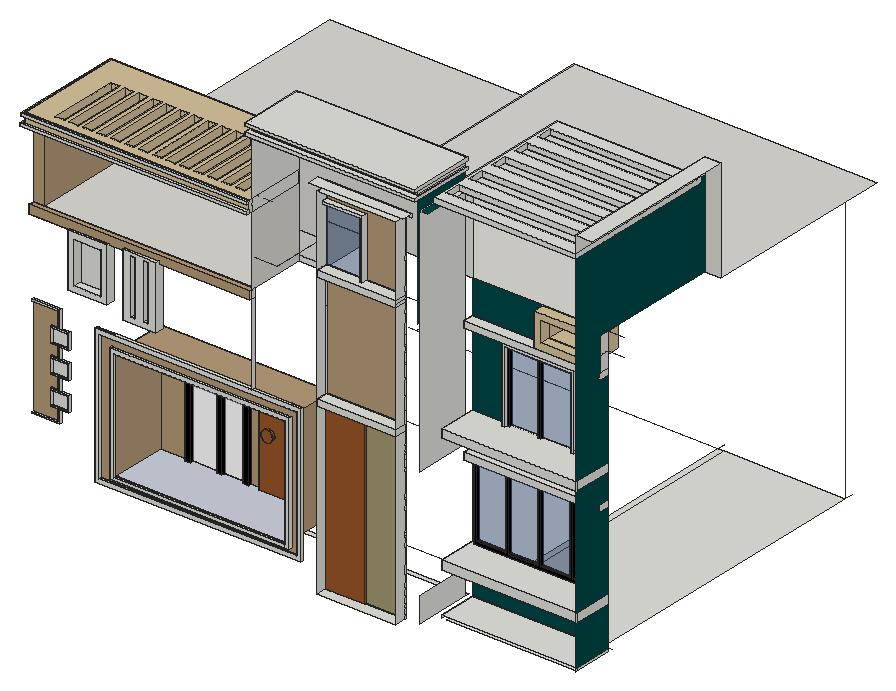
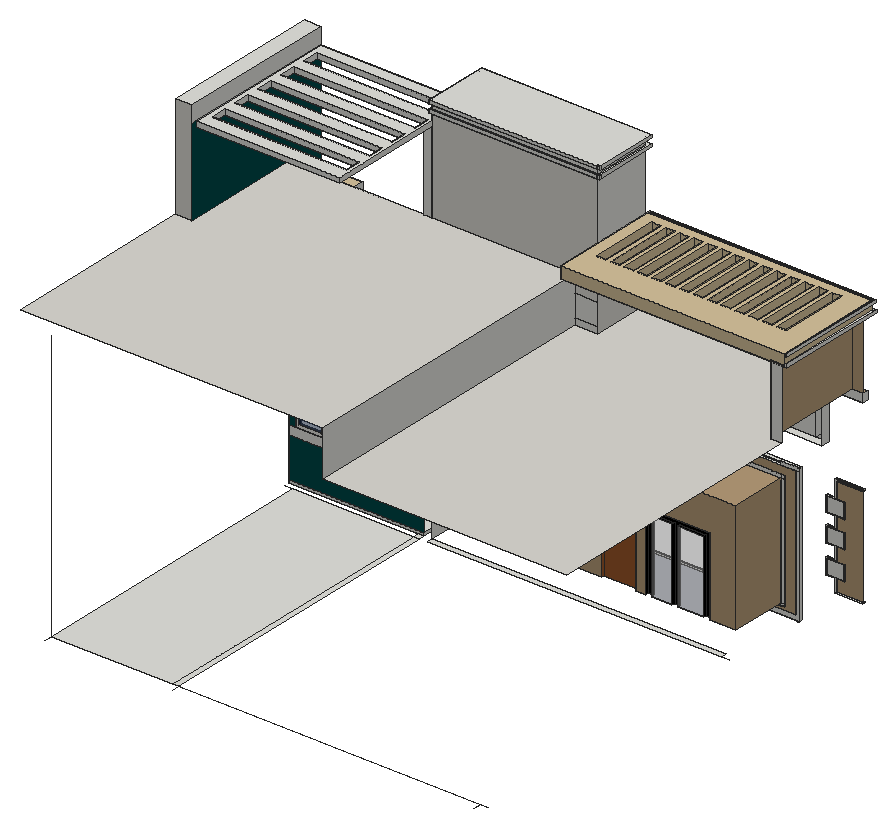
# SketchUp Ruby script. Lengths in inches.
U = 1.inch
M = Sketchup.active_model
def pt(a) = Geom::Point3d.new(a.map { |v| v * U })
def face(e, loops, mat)
  f = e.add_face(loops[0].map { |a| pt(a) })
  loops[1..].each { |l| e.add_face(l.map { |a| pt(a) }).erase! }
  f.material = f.back_material = mat if mat
  f
end
# faces: each face lists its corners as indices into pts; further lists are holes
def faces(e, pts, list, mat = nil) = list.each { |f| face(e, (f[0].is_a?(Array) ? f : [f]).map { |l| l.map { |i| pts[i] } }, mat) }
# xy, xz, yz: faces in a plane at the given z, y or x. An outline is a flat list of corners, or four numbers for a rectangle; further outlines are holes
def ring(l) = l.size == 4 ? [[l[0], l[1]], [l[2], l[1]], [l[2], l[3]], [l[0], l[3]]] : l.each_slice(2).to_a
def flat(e, list, mat, &to3) = list.each { |f| face(e, (f[0].is_a?(Array) ? f : [f]).map { |l| ring(l).map { |u, v| to3.(u, v) } }, mat) }
def xy(e, z, list, mat = nil) = flat(e, list, mat) { |x, y| [x, y, z] }
def xz(e, y, list, mat = nil) = flat(e, list, mat) { |x, z| [x, y, z] }
def yz(e, x, list, mat = nil) = flat(e, list, mat) { |y, z| [x, y, z] }
def lines(e, pts, list) = list.each { |a, b| e.add_line(pt(pts[a]), pt(pts[b])) }
# prism: a flat outline (further loops are holes) pulled along v
def prism(e, loops, v, mat = nil)
  f = face(e, loops, mat); d = Geom::Vector3d.new(v.map { |x| x * U })
  f.pushpull(f.normal.samedirection?(d) ? d.length : -d.length)
end
def box(e, o, s, mat = nil) = prism(e, [[o, [o[0] + s[0], o[1], o[2]], [o[0] + s[0], o[1] + s[1], o[2]], [o[0], o[1] + s[1], o[2]]]], [0, 0, s[2]], mat)
def at(x, y, z, deg = 0) = Geom::Transformation.translation(pt([x, y, z])) * Geom::Transformation.rotation(ORIGIN, Z_AXIS, deg.degrees)
def axes(o, x, y, z) = Geom::Transformation.new([*x, 0, *y, 0, *z, 0, *pt(o).to_a, 1])
def part(name) = M.definitions.add(name)
# library, detail: a bought-in or finely detailed component or shape, given as its bounding box
def library(name, o, s) = part(name).tap { |d| box(d.entities, o, s) }
def detail(e, o, s) = box(e.add_group.entities, o, s)
def put(e, d, t, mat = nil) = e.add_instance(d, t).tap { |i| i.material = mat if mat }
def group(e, t, mat = nil) = e.add_group.tap { |g| g.transformation = t; g.material = mat if mat }.entities
root = M.entities
M.materials.add("[0034_Wheat]").color = [214, 194, 156]
M.materials.add("[0035_Tan]").color = [181, 155, 120]
M.materials.add("[0079_Teal]").color = [0, 71, 71]
M.materials.add("[0137_Black]").color = [0, 0, 0]
M.materials.add("[Marble Carrara Floor Tile]").color = [204, 208, 219]
M.materials.add("[Terrazzo Tile Light]").color = [219, 217, 210]
M.materials.add("[Translucent Glass Blue]").color = [52, 78, 124]
M.materials["[Translucent Glass Blue]"].alpha = 0.5
M.materials.add("[Translucent Glass Gray]").color = [201, 201, 201]
M.materials["[Translucent Glass Gray]"].alpha = 0.5
M.materials.add("[Wood Cherry Original]").color = [152, 86, 42]
M.materials.add("[Wood Lumber ButtJoined]").color = [164, 152, 112]
xy(root,120,[[437.125,271.56,577.1875,313.125],[106.1875,313.125,423.03,319.125],[431.125,313.125,437.125,319.125],[431.125,319.125,437.125,643.9375],[437.125,319.125,568.1875,643.9375]])
xy(root,121,[[323.96,237.8125,409.46,237.8125,409.46,249.8125,366.71,249.8125,366.71,248.8125,323.96,248.8125],[323.96,248.8125,366.71,249.8125],[323.96,249.8125,366.71,250.75],[366.71,249.8125,409.46,250.75]])
xy(root,123,[[431.125,271.56,577.1875,313.125]])
xy(root,136.125,[[74.71,249.8125,296.54,252.8125],[74.71,252.8125,296.54,253.5]])
xy(root,140.43,[[79.1,249.8125,292.23,252.8125]])
xy(root,144.1875,[[91.02,249.8125,284.58,252.8125]])
xy(root,147.125,[[95.27,249.8125,279.28,252.8125]])
xy(root,147.27,[[95.27,252.8125,279.28,252.8125,279.28,313.125,239.67,313.125,239.67,310.125,203.67,310.125,203.67,313.125,192.46,313.125,192.46,310.125,186.46,310.125,186.46,313.125,164.08,313.125,164.08,310.125,158.08,310.125,158.08,313.125,129.71,313.125,129.71,310.125,123.71,310.125,123.71,313.125,95.27,313.125]],"[Marble Carrara Floor Tile]")
xy(root,166.28,[[431.125,271.56,577.1875,313.125]])
xy(root,176.29,[[431.125,271.56,577.1875,271.56,577.1875,313.125,569.6,313.125,569.6,310.125,435.12,310.125,435.12,313.125,431.125,313.125],[435.12,310.125,569.6,313.125]])
xy(root,177.18,[[6.1875,251.5,36.19,253.5]])
xy(root,178.93,[[6.1875,251.5,34.19,253.5]])
xy(root,179.29,[[438.12,310.125,470.05,313.125],[473.05,310.125,503.8,313.125],[506.8,310.125,538.43,313.125],[541.43,310.125,566.6,313.125]],"[0137_Black]")
xy(root,191.55,[[25.74,251.5,34.19,253.5],[36.19,251.5,46.11,253.5]])
xy(root,192.55,[[26.74,251.5,45.11,253.5]])
xy(root,207.43,[[26.74,251.5,45.11,253.5]])
xy(root,208.43,[[25.74,251.5,34.15,253.5],[36.19,251.5,46.11,253.5]])
xy(root,222.43,[[25.74,251.5,34.15,253.5],[36.19,251.5,46.11,253.5]])
xy(root,223.43,[[26.74,251.5,45.11,253.5]])
xy(root,225.27,[[129.71,310.125,158.08,313.125],[164.08,310.125,186.46,313.125]],"[0137_Black]")
xy(root,231.27,[[123.71,310.125,192.46,313.125]],"[0137_Black]")
xy(root,238.3,[[26.74,251.5,45.11,253.5]])
xy(root,239.3,[[25.74,251.5,34.15,253.5],[36.19,251.5,46.11,253.5]])
xy(root,239.64,[[203.67,310.125,239.67,313.125]],"[Wood Cherry Original]")
xy(root,251.74,[[25.74,251.5,34.15,253.5],[36.19,251.5,46.11,253.5]])
xy(root,252.74,[[26.74,251.5,45.11,253.5]])
xy(root,256.41,[[438.12,310.125,470.05,313.125],[473.05,310.125,503.8,313.125],[506.8,310.125,538.43,313.125],[541.43,310.125,566.6,313.125]],"[0137_Black]")
xy(root,259.41,[[431.125,301.125,431.125,313.125,435.12,313.125,435.12,310.125,569.6,310.125,569.6,313.125,577.1875,313.125,577.1875,301.125],[435.12,310.125,569.6,313.125]])
xy(root,267,[[95.27,249.8125,279.28,252.8125],[431.125,301.125,577.1875,313.125]])
xy(root,267,[[95.27,252.8125,279.28,313.125]],"[0035_Tan]")
xy(root,267.61,[[26.74,251.5,45.11,253.5]])
xy(root,268.61,[[25.74,251.5,34.15,253.5],[36.19,251.5,46.11,253.5]])
xy(root,271.125,[[91.02,249.8125,284.58,252.8125]])
xy(root,280.1875,[[79.1,249.8125,292.23,252.8125]])
xy(root,284.3125,[[74.71,249.8125,243.98,249.8125,243.98,253.5,95.27,253.5,95.27,252.8125,74.71,252.8125],[243.98,249.8125,296.54,252.8125],[74.71,252.8125,95.27,253.5]])
xy(root,285.5,[[6.1875,251.5,34.15,253.5]])
xy(root,287.35,[[6.1875,251.5,36.19,253.5]])
xy(root,293.48,[[431.125,271.56,577.1875,313.125]])
xy(root,301.91,[[323.96,237.8125,323.96,248.8125,366.71,248.8125,366.71,250.75,409.46,250.75,409.46,237.8125],[323.96,248.8125,366.71,250.75]])
xy(root,303.01,[[431.125,271.56,577.1875,271.56,577.1875,313.125,545.36,313.125,545.36,307.125,542.36,307.125,542.36,310.125,539.8,310.125,539.8,313.125,507.6,313.125,507.6,310.125,504.6,310.125,504.6,313.125,473.54,313.125,473.54,310.125,470.98,310.125,470.98,307.125,467.98,307.125,467.98,313.125,431.125,313.125],[467.98,307.125,470.98,313.125],[542.36,307.125,545.36,313.125],[470.98,310.125,473.54,313.125],[504.6,310.125,507.6,313.125],
  [539.8,310.125,542.36,313.125]])
xy(root,306.52,[[109.1875,244.5,145.3125,253.5]])
xy(root,308.55,[[323.96,237.8125,409.46,250.75]])
xy(root,312.27,[[118.125,244.5,122.875,253.5],[131.8125,244.5,136,253.5]])
xy(root,314.76,[[50.28,244.5,92.36,253.5]])
xy(root,321.06,[[56.57,244.5,86.07,253.5]])
xy(root,366,[[56.57,244.5,86.07,253.5]])
xy(root,371.77,[[118.125,244.5,122.875,253.5],[131.8125,244.5,136,253.5],[50.28,247.5,92.36,253.5],[145,247.5,145.3125,253.5]])
xy(root,371.77,[[6.1875,247.5,50.28,253.5],[92.36,247.5,109.1875,253.5],[145.3125,247.5,243.98,253.5]],"[0035_Tan]")
xy(root,372.77,[[50.28,244.5,92.36,247.5]])
xy(root,374.77,[[109.1875,244.5,145.3125,247.5]])
xy(root,377.44,[[473.54,310.125,504.6,313.125],[507.6,310.125,539.8,313.125]],"[0137_Black]")
xy(root,380,[[470.98,307.125,542.36,310.125]])
xy(root,380.6875,[[6.1875,247.5,243.98,253.5]],"[0035_Tan]")
xy(root,380.6875,[[17.6875,253.5,243.98,253.5,243.98,313.125,269.04,313.125,269.04,652.9375,6.1875,652.9375,6.1875,363.1875,17.6875,363.1875]],"[Terrazzo Tile Light]")
xy(root,383,[[467.98,307.125,545.36,313.125]])
xy(root,387,[[431.125,301.125,577.1875,313.125]])
xy(root,394.0625,[[431.125,301.125,577.1875,301.125,577.1875,301.875,506.79,301.875,506.79,313.125,431.125,313.125],[506.79,301.875,577.1875,313.125]])
xy(root,401.12,[[513.85,301.875,570.13,313.125],[513.85,313.125,570.13,335.6875]],"[0034_Wheat]")
xy(root,423.19,[[513.85,301.875,570.13,313.125],[513.85,313.125,570.13,335.6875]],"[0034_Wheat]")
xy(root,426.24,[[323.96,237.8125,409.46,250.75]])
xy(root,430.25,[[506.79,301.875,577.1875,313.125]],"[0034_Wheat]")
xy(root,430.25,[[269.04,313.125,577.1875,313.125,577.1875,443.1875,594.5625,443.1875,594.5625,652.9375,269.04,652.9375]],"[Terrazzo Tile Light]")
xy(root,433.05,[[323.96,237.8125,409.46,237.8125,409.46,250.75,367.11,250.75,367.11,244.875,364.11,244.875,364.11,250.75,323.96,250.75],[364.11,244.875,367.11,250.75]])
xy(root,456,[[[0,243.25,243.98,363.1875],[161.16,256.96,170.97,331.71],[26.72,256.96,36.53,331.71],[41.66,256.96,51.47,331.71],[56.6,256.96,66.41,331.71],[71.53,256.96,81.35,331.71],[86.47,256.96,96.28,331.71],[101.41,256.96,111.22,331.71],[116.35,256.96,126.16,331.71],[131.28,256.96,141.1,331.71],[146.22,256.96,156.03,331.71],[176.1,256.96,185.91,331.71],[191.03,256.96,200.85,331.71],[205.97,256.96,215.78,331.71],[220.91,256.96,230.72,331.71]]],"[0034_Wheat]")
xy(root,458.95,[[0,243.25,2.25,246.25],[2.25,243.25,243.98,246.25],[0,246.25,2.25,363.1875]])
xy(root,465.625,[[0.4375,243.25,0.4375,363.1875,2.25,363.1875,2.25,246.25,243.98,246.25,243.98,243.25]])
xy(root,468.57,[[0.4375,243.25,243.98,243.25,243.98,246.25,2.25,246.25,2.25,363.1875,0.4375,363.1875]])
xy(root,468.625,[[[2.25,246.25,243.98,363.1875],[161.16,256.96,170.97,331.71],[26.72,256.96,36.53,331.71],[41.66,256.96,51.47,331.71],[56.6,256.96,66.41,331.71],[71.53,256.96,81.35,331.71],[86.47,256.96,96.28,331.71],[101.41,256.96,111.22,331.71],[116.35,256.96,126.16,331.71],[131.28,256.96,141.1,331.71],[146.22,256.96,156.03,331.71],[176.1,256.96,185.91,331.71],[191.03,256.96,200.85,331.71],[205.97,256.96,215.78,331.71],[220.91,256.96,230.72,331.71]]],"[0034_Wheat]")
xy(root,494.21,[[323.96,244.875,364.11,250.75]])
xy(root,497.21,[[323.96,244.875,367.11,250.75]])
xy(root,509.47,[[323.96,237.8125,409.46,249.8125]])
xy(root,514.78,[[315.58,237.8125,416.24,249.8125],[323.96,249.8125,409.46,250.75]])
xy(root,518.125,[[[422.6875,270.3125,422.6875,438.125,577.1875,438.125,577.1875,270.3125,431.125,270.3125,431.125,283.49,570.77,283.49,570.77,300.68,431.125,300.68,431.125,313.125,423.03,313.125,423.03,270.3125],[426.33,314.3,570.77,331.49],[426.33,345.12,570.77,362.3],[426.33,375.93,570.77,393.12],[426.33,406.74,570.77,423.93]],[423.03,270.3125,431.125,270.3125,431.125,283.49,426.33,283.49,426.33,300.68,431.125,300.68,431.125,313.125,423.03,313.125],[426.33,283.49,431.125,300.68]])
xy(root,518.125,[[423.03,252.8125,431.125,270.3125]],"[0079_Teal]")
xy(root,523.8125,[[[422.6875,270.3125,577.1875,438.125],[426.33,283.49,570.77,300.68],[426.33,314.3,570.77,331.49],[426.33,345.12,570.77,362.3],[426.33,375.93,570.77,393.12],[426.33,406.74,570.77,423.93]]])
xy(root,531.41,[[241.23,243.8125,241.23,313.125,243.98,313.125,243.98,249.8125,423.03,249.8125,423.03,313.125,243.98,313.125,243.98,314.6875,425.03,314.6875,425.03,243.8125],[241.23,313.125,243.98,314.6875]])
xy(root,534.9375,[[241.23,243.8125,425.03,243.8125,425.03,314.6875,243.98,314.6875,243.98,313.125,423.03,313.125,423.03,249.8125,243.98,249.8125,243.98,313.125,241.23,313.125],[241.23,313.125,243.98,314.6875]])
xy(root,540.18,[[241.23,243.8125,241.23,313.125,243.98,313.125,243.98,249.8125,423.03,249.8125,423.03,313.125,243.98,313.125,243.98,314.5625,425.03,314.5625,425.03,243.8125],[241.23,313.125,243.98,314.5625]])
xy(root,541.5625,[[577.1875,270.3125,594.5625,443.1875]])
xy(root,543.75,[[241.23,243.8125,425.03,243.8125,425.03,314.5625,243.98,314.5625,243.98,313.125,241.23,313.125],[241.23,313.125,243.98,314.5625]])
xz(root,237.8125,[[323.96,301.91,409.46,308.55],[323.96,426.24,409.46,433.05]])
xz(root,243.25,[[0,456,243.98,458.95],[0.4375,465.625,243.98,468.57]])
xz(root,243.8125,[[241.23,531.41,425.03,534.9375],[241.23,540.18,425.03,543.75]])
xz(root,244.5,[[[109.1875,306.52,145.3125,374.77],[118.125,312.27,122.875,371.77],[131.8125,312.27,136,371.77]],[[50.28,314.76,92.36,372.77],[56.57,321.06,86.07,366]]])
xz(root,244.875,[[364.11,433.05,367.11,433.05,367.11,497.21,323.96,497.21,323.96,494.21,364.11,494.21]])
xz(root,246.25,[[2.25,465.625,243.98,468.57],[2.25,468.57,243.98,468.625]])
xz(root,246.25,[[2.25,458.95,243.98,465.625]],"[0034_Wheat]")
xz(root,247.5,[[50.28,371.77,92.36,372.77]])
xz(root,247.5,[[6.1875,371.77,50.28,371.77,50.28,372.77,92.36,372.77,92.36,371.77,109.1875,371.77,109.1875,374.77,145.3125,374.77,145.3125,371.77,243.98,371.77,243.98,380.6875,6.1875,380.6875]],"[0035_Tan]")
xz(root,248.8125,[[323.96,121,366.71,301.91]],"[Wood Cherry Original]")
xz(root,249.8125,[[[74.71,136.125,296.54,284.3125],[79.1,140.43,292.23,280.1875]],[[91.02,144.1875,284.58,271.125],[95.27,147.125,279.28,267]],[323.96,509.47,409.46,514.78],[409.46,510.78,416.24,514.78],[243.98,531.37,423.03,531.41],
  [243.98,531.41,423.03,534.9375],[243.98,534.9375,423.03,540.18]])
xz(root,250.75,[[323.96,121,366.71,301.91],[323.96,301.91,409.46,308.55],[323.96,426.24,409.46,429.68],[323.96,429.68,323.96,430.05,367.11,430.05,367.11,433.05,409.46,433.05,409.46,429.68],[320.96,430.05,323.96,497.21],
  [323.96,430.05,367.11,433.05]])
xz(root,250.75,[[323.96,308.55,409.46,426.24],[367.11,433.05,409.46,433.05,409.46,514.78,323.96,514.78,323.96,497.21,367.11,497.21]],"[0035_Tan]")
xz(root,250.75,[[323.96,433.05,364.11,494.21]],"[Translucent Glass Blue]")
xz(root,250.75,[[366.71,121,409.46,301.91]],"[Wood Lumber ButtJoined]")
xz(root,251.5,[[6.1875,177.18,36.19,177.18,36.19,191.55,34.19,191.55,34.19,178.93,6.1875,178.93],[[25.74,191.55,46.11,208.43],[26.74,192.55,45.11,207.43]],[34.15,208.43,36.19,222.43],[[25.74,222.43,46.11,239.3],[26.74,223.43,45.11,238.3]],[34.15,239.3,36.19,251.74],
  [[25.74,251.74,46.11,268.61],[26.74,252.74,45.11,267.61]],[34.15,268.61,36.19,268.61,36.19,287.35,6.1875,287.35,6.1875,285.5,34.15,285.5]])
xz(root,252.8125,[[74.71,136.125,296.54,136.125,296.54,139.43,292.23,139.43,292.23,140.43,79.1,140.43,79.1,280.1875,74.71,280.1875],[292.23,139.43,296.54,147.27],[91.02,144.1875,95.27,145.0625],[95.27,144.1875,279.28,145.0625],[279.28,144.1875,284.58,147.27],
  [91.02,145.0625,95.27,147.125],[95.27,145.0625,279.28,147.125],[91.02,147.125,95.27,267],[95.27,147.125,279.28,147.27],[279.28,147.27,284.58,267],
  [292.23,147.27,296.54,267],[91.02,267,95.27,271.125],[95.27,267,284.58,271.125],[292.23,267,296.54,280.1875],[74.71,280.1875,95.27,284.3125],
  [284.58,280.1875,296.54,284.3125]])
xz(root,252.8125,[[[79.1,140.43,292.23,280.1875],[91.02,144.1875,284.58,271.125]]],"[0035_Tan]")
xz(root,253.5,[[26.74,192.55,45.11,207.43],[26.74,223.43,45.11,238.3],[26.74,252.74,45.11,267.61],[109.1875,312.27,118.125,371.77],[118.125,312.27,122.875,371.77],
  [122.875,312.27,131.8125,371.77],[131.8125,312.27,136,371.77],[136,312.27,145,371.77],[56.57,321.06,86.07,366],[6.1875,371.77,6.1875,380.6875,243.98,380.6875,243.98,371.77,92.36,371.77,92.36,372.29,50.28,372.29,50.28,371.77],
  [50.28,371.77,92.36,372.29]])
xz(root,253.5,[[6.1875,178.93,34.19,178.93,34.19,191.55,25.74,191.55,25.74,208.43,34.15,208.43,34.15,222.43,25.74,222.43,25.74,239.3,34.15,239.3,34.15,251.74,25.74,251.74,25.74,268.61,34.15,268.61,34.15,285.5,6.1875,285.5],[6.1875,380.6875,17.6875,456.625]],"[0035_Tan]")
xz(root,256.96,[[26.72,456,36.53,468.625],[41.66,456,51.47,468.625],[56.6,456,66.41,468.625],[71.53,456,81.35,468.625],[86.47,456,96.28,468.625],
  [101.41,456,111.22,468.625],[116.35,456,126.16,468.625],[131.28,456,141.1,468.625],[146.22,456,156.03,468.625],[161.16,456,170.97,468.625],
  [176.1,456,185.91,468.625],[191.03,456,200.85,468.625],[205.97,456,215.78,468.625],[220.91,456,230.72,468.625]],"[0034_Wheat]")
xz(root,270.3125,[[422.6875,518.125,577.1875,523.8125]])
xz(root,271.56,[[431.125,166.28,577.1875,176.29],[431.125,293.48,577.1875,303.01]])
xz(root,283.49,[[426.33,518.125,570.77,523.8125]])
xz(root,300.68,[[426.33,518.125,570.77,523.8125]])
xz(root,301.125,[[431.125,259.41,577.1875,267],[431.125,387,577.1875,394.0625]])
xz(root,301.875,[[[506.79,394.0625,577.1875,430.25],[513.85,401.12,570.13,423.19]]],"[0034_Wheat]")
xz(root,307.125,[[467.98,303.01,470.98,303.01,470.98,380,542.36,380,542.36,303.01,545.36,303.01,545.36,383,467.98,383]])
xz(root,307.125,[[214.3,197.28,215.89,197.49,217.36,198.1,218.63,199.07,219.61,200.34,220.22,201.82,220.43,203.41,220.22,204.99,219.61,206.47,218.63,207.74,217.36,208.71,215.89,209.32,214.3,209.53,212.72,209.32,211.24,208.71,209.97,207.74,209,206.47,208.39,204.99,208.18,203.41,208.39,201.82,209,200.34,209.97,199.07,211.24,198.1,212.72,197.49]],"[Wood Cherry Original]")
xz(root,310.125,[[123.71,147.27,129.71,147.27,129.71,225.27,158.08,225.27,158.08,147.27,164.08,147.27,164.08,225.27,186.46,225.27,186.46,147.27,192.46,147.27,192.46,231.27,123.71,231.27],[[435.12,176.29,569.6,259.41],[438.12,179.29,470.05,256.41],[506.8,179.29,538.43,256.41],[473.05,179.29,503.8,256.41],[541.43,179.29,566.6,256.41]],[470.98,303.01,473.54,303.01,473.54,377.44,504.6,377.44,504.6,303.01,507.6,303.01,507.6,377.44,539.8,377.44,539.8,303.01,542.36,303.01,542.36,380,470.98,380]],"[0137_Black]")
xz(root,310.125,[[[203.67,147.27,239.67,239.64],[214.3,197.28,212.72,197.49,211.24,198.1,209.97,199.07,209,200.34,208.39,201.82,208.18,203.41,208.39,204.99,209,206.47,209.97,207.74,211.24,208.71,212.72,209.32,214.3,209.53,215.89,209.32,217.36,208.71,218.63,207.74,219.61,206.47,220.22,204.99,220.43,203.41,220.22,201.82,219.61,200.34,218.63,199.07,217.36,198.1,215.89,197.49]]],"[Wood Cherry Original]")
xz(root,313.125,[[431.125,120,577.1875,123],[431.125,166.28,577.1875,176.29],[[435.12,176.29,569.6,259.41],[438.12,179.29,470.05,256.41],[506.8,179.29,538.43,256.41],[473.05,179.29,503.8,256.41],[541.43,179.29,566.6,256.41]],[431.125,259.41,577.1875,267],[431.125,293.48,577.1875,303.01],
  [571.72,303.01,577.1875,387],[243.98,380.6875,269.04,387],[243.98,387,269.04,411],[431.125,387,577.1875,394.0625],[[506.79,394.0625,577.1875,430.25],[513.85,401.12,570.13,423.19]],
  [423.03,430.25,431.125,518.125],[241.23,531.41,243.98,534.9375],[243.98,531.41,423.03,534.9375],[243.98,534.9375,423.03,540.18],[241.23,540.18,243.98,543.75]])
xz(root,313.125,[[95.27,147.27,123.71,147.27,123.71,231.27,192.46,231.27,192.46,147.27,203.67,147.27,203.67,239.64,239.67,239.64,239.67,147.27,279.28,147.27,279.28,267,95.27,267]],"[0035_Tan]")
xz(root,313.125,[[431.125,123,577.1875,166.28],[431.125,176.29,435.12,259.41],[569.6,176.29,577.1875,259.41],[431.125,267,577.1875,293.48],[431.125,303.01,467.98,303.01,467.98,383,545.36,383,545.36,303.01,571.72,303.01,571.72,387,431.125,387],
  [431.125,394.0625,506.79,430.25]],"[0079_Teal]")
xz(root,313.125,[[243.98,411,243.98,531.41,423.03,531.41,423.03,430.25,269.04,430.25,269.04,411]],"[Terrazzo Tile Light]")
xz(root,313.125,[[438.12,179.29,470.05,256.41],[473.05,179.29,503.8,256.41],[506.8,179.29,538.43,256.41],[541.43,179.29,566.6,256.41],[473.54,303.01,504.6,377.44],
  [507.6,303.01,539.8,377.44]],"[Translucent Glass Blue]")
xz(root,313.125,[[129.71,147.27,158.08,225.27],[164.08,147.27,186.46,225.27]],"[Translucent Glass Gray]")
xz(root,314.3,[[426.33,518.125,570.77,523.8125]])
xz(root,314.5625,[[241.23,540.18,243.98,543.75],[243.98,540.18,425.03,543.75]])
xz(root,314.6875,[[241.23,531.41,243.98,534.9375],[243.98,531.41,425.03,534.9375]])
xz(root,331.49,[[426.33,518.125,570.77,523.8125]])
xz(root,331.71,[[26.72,456,36.53,468.625],[41.66,456,51.47,468.625],[56.6,456,66.41,468.625],[71.53,456,81.35,468.625],[86.47,456,96.28,468.625],
  [101.41,456,111.22,468.625],[116.35,456,126.16,468.625],[131.28,456,141.1,468.625],[146.22,456,156.03,468.625],[161.16,456,170.97,468.625],
  [176.1,456,185.91,468.625],[191.03,456,200.85,468.625],[205.97,456,215.78,468.625],[220.91,456,230.72,468.625]],"[0034_Wheat]")
xz(root,335.6875,[[513.85,401.12,570.13,423.19]],"[0034_Wheat]")
xz(root,345.12,[[426.33,518.125,570.77,523.8125]])
xz(root,362.3,[[426.33,518.125,570.77,523.8125]])
xz(root,363.1875,[[6.1875,380.6875,17.6875,456],[0,456,2.25,458.95],[2.25,456,17.6875,456.625],[0.4375,465.625,2.25,468.57]])
xz(root,363.1875,[[17.6875,456,17.6875,456.625,2.25,456.625,2.25,468.625,243.98,468.625,243.98,456]],"[0034_Wheat]")
xz(root,375.93,[[426.33,518.125,570.77,523.8125]])
xz(root,393.12,[[426.33,518.125,570.77,523.8125]])
xz(root,406.74,[[426.33,518.125,570.77,523.8125]])
xz(root,423.93,[[426.33,518.125,570.77,523.8125]])
xz(root,438.125,[[422.6875,518.125,577.1875,523.8125]])
xz(root,443.1875,[[577.1875,430.25,594.5625,541.5625]],"[Terrazzo Tile Light]")
yz(root,0,[[243.25,456,363.1875,458.95]])
yz(root,0.4375,[[243.25,465.625,363.1875,468.57]])
yz(root,2.25,[[246.25,465.625,363.1875,468.57],[246.25,468.57,363.1875,468.625]])
yz(root,2.25,[[246.25,458.95,363.1875,465.625]],"[0034_Wheat]")
yz(root,6.1875,[[247.5,371.77,253.5,380.6875]])
yz(root,17.6875,[[253.5,380.6875,363.1875,456.625]],"[0035_Tan]")
yz(root,25.74,[[251.5,191.55,253.5,208.43],[251.5,222.43,253.5,239.3],[251.5,251.74,253.5,268.61]])
yz(root,26.72,[[256.96,456,331.71,468.625]],"[0034_Wheat]")
yz(root,26.74,[[251.5,192.55,253.5,207.43],[251.5,223.43,253.5,238.3],[251.5,252.74,253.5,267.61]])
yz(root,34.15,[[251.5,208.43,253.5,222.43],[251.5,239.3,253.5,251.74],[251.5,268.61,253.5,285.5]])
yz(root,34.19,[[251.5,178.93,253.5,191.55]])
yz(root,36.19,[[251.5,177.18,253.5,191.55],[251.5,208.43,253.5,222.43],[251.5,239.3,253.5,251.74],[251.5,268.61,253.5,287.35]])
yz(root,36.53,[[256.96,456,331.71,468.625]],"[0034_Wheat]")
yz(root,41.66,[[256.96,456,331.71,468.625]],"[0034_Wheat]")
yz(root,45.11,[[251.5,192.55,253.5,207.43],[251.5,223.43,253.5,238.3],[251.5,252.74,253.5,267.61]])
yz(root,46.11,[[251.5,191.55,253.5,208.43],[251.5,222.43,253.5,239.3],[251.5,251.74,253.5,268.61]])
yz(root,50.28,[[244.5,314.76,244.5,372.77,247.5,372.77,247.5,371.77,253.5,371.77,253.5,314.76]])
yz(root,51.47,[[256.96,456,331.71,468.625]],"[0034_Wheat]")
yz(root,56.57,[[244.5,321.06,253.5,366]])
yz(root,56.6,[[256.96,456,331.71,468.625]],"[0034_Wheat]")
yz(root,66.41,[[256.96,456,331.71,468.625]],"[0034_Wheat]")
yz(root,71.53,[[256.96,456,331.71,468.625]],"[0034_Wheat]")
yz(root,74.71,[[249.8125,136.125,252.8125,284.3125],[252.8125,136.125,253.5,280.1875],[252.8125,280.1875,253.5,284.3125]])
yz(root,79.1,[[249.8125,140.43,252.8125,280.1875]])
yz(root,81.35,[[256.96,456,331.71,468.625]],"[0034_Wheat]")
yz(root,86.07,[[244.5,321.06,253.5,366]])
yz(root,86.47,[[256.96,456,331.71,468.625]],"[0034_Wheat]")
yz(root,91.02,[[249.8125,144.1875,252.8125,271.125]])
yz(root,92.36,[[244.5,314.76,253.5,314.76,253.5,371.77,247.5,371.77,247.5,372.77,244.5,372.77]])
yz(root,95.27,[[249.8125,147.125,252.8125,267]])
yz(root,95.27,[[252.8125,147.27,313.125,267]],"[0035_Tan]")
yz(root,96.28,[[256.96,456,331.71,468.625]],"[0034_Wheat]")
yz(root,101.41,[[256.96,456,331.71,468.625]],"[0034_Wheat]")
yz(root,109.1875,[[244.5,306.52,244.5,374.77,247.5,374.77,247.5,371.77,253.5,371.77,253.5,306.52]])
yz(root,111.22,[[256.96,456,331.71,468.625]],"[0034_Wheat]")
yz(root,116.35,[[256.96,456,331.71,468.625]],"[0034_Wheat]")
yz(root,118.125,[[244.5,312.27,253.5,371.77]])
yz(root,122.875,[[244.5,312.27,253.5,371.77]])
yz(root,123.71,[[310.125,147.27,313.125,231.27]])
yz(root,126.16,[[256.96,456,331.71,468.625]],"[0034_Wheat]")
yz(root,129.71,[[310.125,147.27,313.125,225.27]],"[0137_Black]")
yz(root,131.28,[[256.96,456,331.71,468.625]],"[0034_Wheat]")
yz(root,131.8125,[[244.5,312.27,253.5,371.77]])
yz(root,136,[[244.5,312.27,253.5,371.77]])
yz(root,141.1,[[256.96,456,331.71,468.625]],"[0034_Wheat]")
yz(root,145.3125,[[244.5,306.52,253.5,306.52,253.5,371.77,247.5,371.77,247.5,374.77,244.5,374.77]])
yz(root,146.22,[[256.96,456,331.71,468.625]],"[0034_Wheat]")
yz(root,156.03,[[256.96,456,331.71,468.625]],"[0034_Wheat]")
yz(root,158.08,[[310.125,147.27,313.125,225.27]],"[0137_Black]")
yz(root,161.16,[[256.96,456,331.71,468.625]],"[0034_Wheat]")
yz(root,164.08,[[310.125,147.27,313.125,225.27]],"[0137_Black]")
yz(root,170.97,[[256.96,456,331.71,468.625]],"[0034_Wheat]")
yz(root,176.1,[[256.96,456,331.71,468.625]],"[0034_Wheat]")
yz(root,185.91,[[256.96,456,331.71,468.625]],"[0034_Wheat]")
yz(root,186.46,[[310.125,147.27,313.125,225.27]],"[0137_Black]")
yz(root,191.03,[[256.96,456,331.71,468.625]],"[0034_Wheat]")
yz(root,192.46,[[310.125,147.27,313.125,231.27]],"[0137_Black]")
yz(root,200.85,[[256.96,456,331.71,468.625]],"[0034_Wheat]")
yz(root,203.67,[[310.125,147.27,313.125,239.64]],"[Wood Cherry Original]")
yz(root,205.97,[[256.96,456,331.71,468.625]],"[0034_Wheat]")
yz(root,215.78,[[256.96,456,331.71,468.625]],"[0034_Wheat]")
yz(root,220.91,[[256.96,456,331.71,468.625]],"[0034_Wheat]")
yz(root,230.72,[[256.96,456,331.71,468.625]],"[0034_Wheat]")
yz(root,239.67,[[310.125,147.27,313.125,239.64]],"[Wood Cherry Original]")
yz(root,241.23,[[243.8125,531.41,313.125,534.9375],[313.125,531.41,314.6875,534.9375],[243.8125,540.18,313.125,543.75],[313.125,540.18,314.5625,543.75]])
yz(root,243.98,[[249.8125,284.3125,253.5,371.77],[247.5,371.77,249.8125,380.6875],[249.8125,371.77,253.5,380.6875],[243.25,456,246.25,458.95],[246.25,456,249.8125,468.625],
  [249.8125,456,313.125,468.625],[243.25,465.625,246.25,468.57],[249.8125,468.625,313.125,531.41],[249.8125,531.41,313.125,534.9375],[313.125,531.41,314.6875,534.9375],
  [249.8125,534.9375,313.125,540.18],[313.125,540.18,314.5625,543.75]])
yz(root,243.98,[[313.125,456,363.1875,468.625]],"[0034_Wheat]")
yz(root,243.98,[[249.8125,380.6875,313.125,456]],"[Terrazzo Tile Light]")
yz(root,269.04,[[313.125,380.6875,652.9375,430.25]])
yz(root,279.28,[[249.8125,147.125,252.8125,267]])
yz(root,279.28,[[252.8125,147.27,313.125,267]],"[0035_Tan]")
yz(root,284.58,[[249.8125,144.1875,252.8125,271.125]])
yz(root,292.23,[[249.8125,140.43,252.8125,280.1875]])
yz(root,296.54,[[249.8125,136.125,252.8125,284.3125]])
yz(root,323.96,[[237.8125,121,248.8125,301.91],[248.8125,121,249.8125,301.91],[249.8125,121,250.75,301.91],[237.8125,301.91,249.8125,308.55],[249.8125,301.91,250.75,308.55],
  [237.8125,308.55,249.8125,426.24],[249.8125,308.55,250.75,426.24],[237.8125,426.24,249.8125,429.68],[249.8125,426.24,250.75,429.68],[237.8125,429.68,249.8125,433.05],
  [249.8125,429.68,250.75,433.05],[237.8125,433.05,249.8125,433.05,249.8125,494.21,244.875,494.21,244.875,497.21,249.8125,497.21,249.8125,509.47,237.8125,509.47],[249.8125,433.05,250.75,494.21],[244.875,494.21,249.8125,497.21],[249.8125,494.21,250.75,497.21],
  [249.8125,497.21,250.75,514.78]])
yz(root,364.11,[[244.875,433.05,250.75,494.21]])
yz(root,366.71,[[248.8125,121,250.75,301.91]],"[Wood Cherry Original]")
yz(root,367.11,[[244.875,433.05,250.75,497.21]])
yz(root,409.46,[[237.8125,121,249.8125,301.91],[249.8125,121,250.75,301.91],[237.8125,301.91,249.8125,308.55],[249.8125,301.91,250.75,308.55],[237.8125,308.55,249.8125,426.24],
  [249.8125,308.55,250.75,426.24],[237.8125,426.24,249.8125,429.68],[249.8125,426.24,250.75,429.68],[237.8125,429.68,249.8125,433.05],[249.8125,429.68,250.75,433.05],
  [237.8125,433.05,249.8125,509.47],[249.8125,433.05,250.75,514.78]])
yz(root,422.6875,[[270.3125,518.125,438.125,523.8125]])
yz(root,423.03,[[252.8125,120,313.125,147.27],[252.8125,267,313.125,518.125],[249.8125,531.41,313.125,534.9375],[249.8125,534.9375,313.125,540.18]])
yz(root,423.03,[[249.8125,411,252.8125,411,252.8125,518.125,313.125,518.125,313.125,531.41,249.8125,531.41]],"[0079_Teal]")
yz(root,425.03,[[243.8125,531.41,314.6875,534.9375],[243.8125,540.18,314.5625,543.75]])
yz(root,426.33,[[283.49,518.125,300.68,523.8125],[314.3,518.125,331.49,523.8125],[345.12,518.125,362.3,523.8125],[375.93,518.125,393.12,523.8125],[406.74,518.125,423.93,523.8125]])
yz(root,431.125,[[271.56,120,313.125,123],[271.56,166.28,313.125,176.29],[301.125,259.41,313.125,267],[271.56,293.48,313.125,303.01],[301.125,387,313.125,394.0625]])
yz(root,435.12,[[310.125,176.29,313.125,259.41]])
yz(root,438.12,[[310.125,179.29,313.125,256.41]],"[0137_Black]")
yz(root,467.98,[[307.125,303.01,313.125,305.62],[307.125,305.62,313.125,383]])
yz(root,470.05,[[310.125,179.29,313.125,256.41]],"[0137_Black]")
yz(root,470.98,[[307.125,303.01,310.125,380]])
yz(root,473.05,[[310.125,179.29,313.125,256.41]],"[0137_Black]")
yz(root,473.54,[[310.125,303.01,313.125,377.44]],"[0137_Black]")
yz(root,503.8,[[310.125,179.29,313.125,256.41]],"[0137_Black]")
yz(root,504.6,[[310.125,303.01,313.125,377.44]],"[0137_Black]")
yz(root,506.79,[[301.875,394.0625,313.125,430.25]])
yz(root,506.8,[[310.125,179.29,313.125,256.41]],"[0137_Black]")
yz(root,507.6,[[310.125,303.01,313.125,377.44]],"[0137_Black]")
yz(root,513.85,[[301.875,401.12,313.125,423.19],[313.125,401.12,335.6875,423.19]],"[0034_Wheat]")
yz(root,538.43,[[310.125,179.29,313.125,256.41]],"[0137_Black]")
yz(root,539.8,[[310.125,303.01,313.125,377.44]],"[0137_Black]")
yz(root,541.43,[[310.125,179.29,313.125,256.41]],"[0137_Black]")
yz(root,542.36,[[307.125,303.01,310.125,380]])
yz(root,545.36,[[307.125,303.01,313.125,305.62],[307.125,305.62,313.125,383]])
yz(root,566.6,[[310.125,179.29,313.125,256.41]],"[0137_Black]")
yz(root,569.6,[[310.125,176.29,313.125,259.41]])
yz(root,570.13,[[301.875,401.12,313.125,423.19],[313.125,401.12,335.6875,423.19]],"[0034_Wheat]")
yz(root,570.77,[[283.49,518.125,300.68,523.8125],[314.3,518.125,331.49,523.8125],[345.12,518.125,362.3,523.8125],[375.93,518.125,393.12,523.8125],[406.74,518.125,423.93,523.8125]])
yz(root,577.1875,[[270.3125,120,271.56,123],[271.56,120,313.125,123],[270.3125,166.28,271.56,176.29],[271.56,166.28,313.125,176.29],[301.125,259.41,313.125,267],
  [270.3125,293.48,271.56,303.01],[271.56,293.48,313.125,303.01],[301.125,387,313.125,394.0625],[301.875,394.0625,313.125,411],[301.875,411,313.125,430.25],
  [270.3125,518.125,438.125,523.8125],[270.3125,523.8125,443.1875,541.5625]])
yz(root,577.1875,[[270.3125,123,313.125,166.28],[270.3125,176.29,270.3125,293.48,313.125,293.48,313.125,267,301.125,267,301.125,259.41,313.125,259.41,313.125,176.29],[270.3125,303.01,270.3125,518.125,438.125,518.125,438.125,523.8125,443.1875,523.8125,443.1875,430.25,301.875,430.25,301.875,394.0625,301.125,394.0625,301.125,387,313.125,387,313.125,303.01]],"[0079_Teal]")
p = [[212.72,310.125,197.49],[214.3,310.125,197.28],[214.3,307.125,197.28],[212.72,307.125,197.49],[215.89,310.125,197.49],[215.89,307.125,197.49],
  [211.24,310.125,198.1],[211.24,307.125,198.1],[217.36,310.125,198.1],[217.36,307.125,198.1],[209.97,310.125,199.07],[209.97,307.125,199.07],
  [218.63,310.125,199.07],[218.63,307.125,199.07],[209,310.125,200.34],[209,307.125,200.34],[219.61,310.125,200.34],[219.61,307.125,200.34],
  [208.39,310.125,201.82],[208.39,307.125,201.82],[220.22,310.125,201.82],[220.22,307.125,201.82],[208.18,310.125,203.41],[208.18,307.125,203.41],
  [220.43,310.125,203.41],[220.43,307.125,203.41],[208.39,310.125,204.99],[208.39,307.125,204.99],[220.22,310.125,204.99],[220.22,307.125,204.99],
  [209,310.125,206.47],[209,307.125,206.47],[219.61,310.125,206.47],[219.61,307.125,206.47],[209.97,310.125,207.74],[209.97,307.125,207.74],
  [218.63,310.125,207.74],[218.63,307.125,207.74],[211.24,310.125,208.71],[211.24,307.125,208.71],[217.36,310.125,208.71],[217.36,307.125,208.71],
  [212.72,310.125,209.32],[212.72,307.125,209.32],[215.89,310.125,209.32],[215.89,307.125,209.32],[214.3,310.125,209.53],[214.3,307.125,209.53],
  [568.1875,643.9375,120],[568.1875,643.9375,411],[431.125,643.9375,120],[431.125,652.9375,120],[106.1875,643.9375,120],[106.1875,652.9375,120],
  [568.1875,652.9375,120],[568.1875,319.125,120],[577.1875,319.125,120],[577.1875,313.125,411],[594.5625,313.125,411],[423.03,313.125,387],
  [269.04,313.125,387],[106.1875,319.125,120],[97.1875,319.125,120],[97.1875,643.9375,120],[423.03,313.125,267],[279.28,313.125,267],
  [423.03,313.125,147.27],[279.28,313.125,147.27],[279.28,252.8125,145.0625],[279.28,249.8125,145.0625],[269.04,252.8125,411],[243.98,252.8125,411],
  [269.04,313.125,411],[243.98,256.96,468.625],[245.66,256.96,468.625],[250.78,256.96,468.625],[260.6,256.96,468.625],[2.25,246.25,456],
  [2.25,246.25,458.95],[243.98,249.8125,540.18],[243.98,249.8125,543.75],[423.03,249.8125,540.18],[423.03,249.8125,543.75],[423.03,313.125,540.18],
  [423.03,313.125,543.75],[577.1875,313.125,430.25],[594.5625,313.125,430.25]]
faces(root,p,[[0,1,2,3],[1,4,5,2],[6,0,3,7],[4,8,9,5],[10,6,7,11],[8,12,13,9],[14,10,11,15],[12,16,17,13],
  [18,14,15,19],[16,20,21,17],[22,18,19,23],[20,24,25,21],[26,22,23,27],[24,28,29,25],[30,26,27,31],[28,32,33,29],
  [34,30,31,35],[32,36,37,33],[38,34,35,39],[36,40,41,37],[42,38,39,43],[40,44,45,41],[46,42,43,47],[44,46,47,45]],"[Wood Cherry Original]")
lines(root,p,[[48,49],[50,51],[52,53],[48,54],[55,56],[57,58],[59,60],[50,52],[61,62],[52,63],[64,65],[66,67],
  [68,69],[70,71],[72,70],[73,74],[75,76],[77,78],[79,80],[81,82],[83,84],[85,86]])
